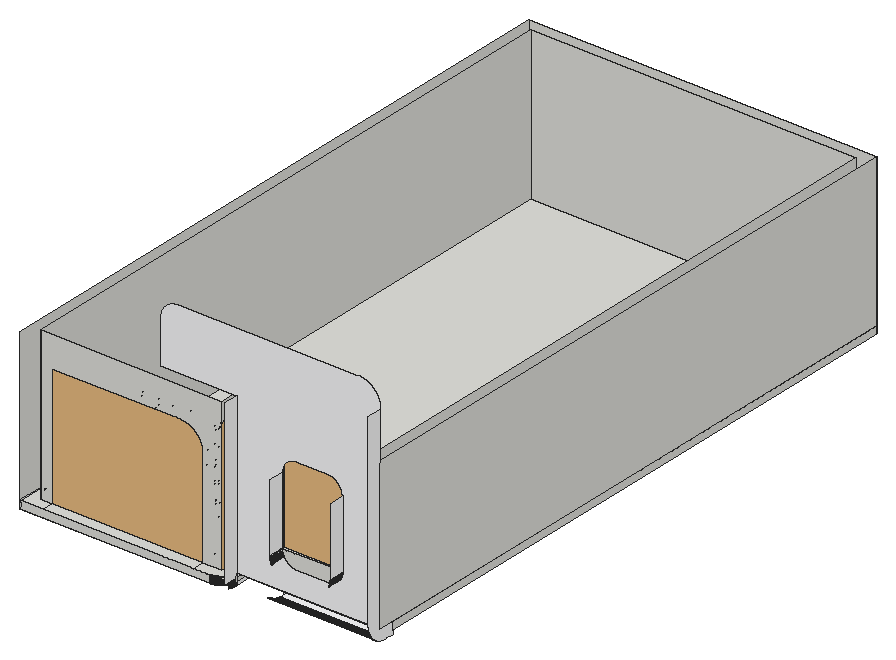
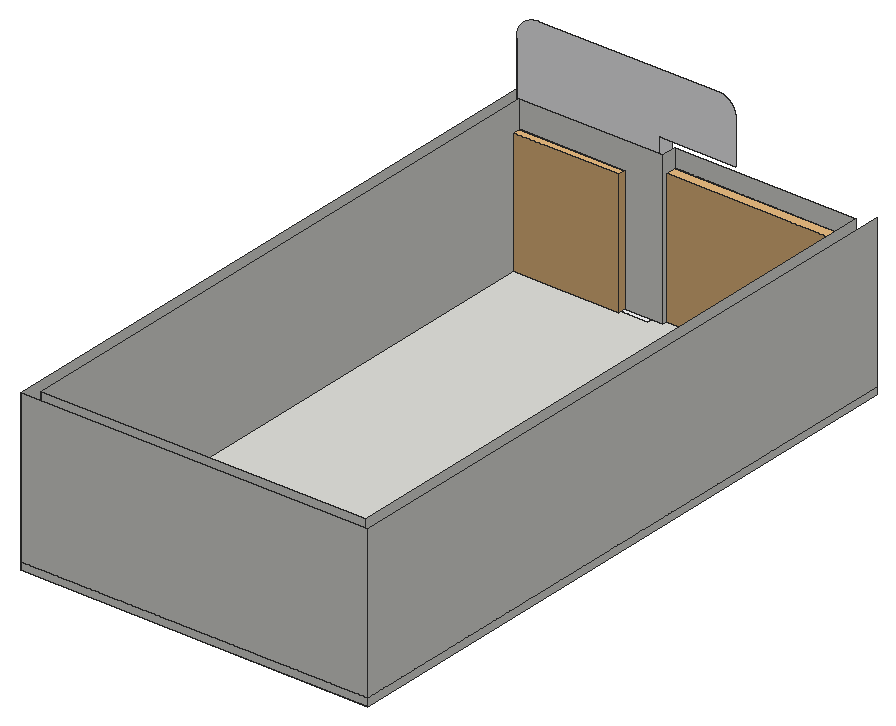
# SketchUp Ruby script. Lengths in inches.
U = 1.inch
M = Sketchup.active_model
def pt(a) = Geom::Point3d.new(a.map { |v| v * U })
def face(e, loops, mat)
  f = e.add_face(loops[0].map { |a| pt(a) })
  loops[1..].each { |l| e.add_face(l.map { |a| pt(a) }).erase! }
  f.material = f.back_material = mat if mat
  f
end
# faces: each face lists its corners as indices into pts; further lists are holes
def faces(e, pts, list, mat = nil) = list.each { |f| face(e, (f[0].is_a?(Array) ? f : [f]).map { |l| l.map { |i| pts[i] } }, mat) }
# xy, xz, yz: faces in a plane at the given z, y or x. An outline is a flat list of corners, or four numbers for a rectangle; further outlines are holes
def ring(l) = l.size == 4 ? [[l[0], l[1]], [l[2], l[1]], [l[2], l[3]], [l[0], l[3]]] : l.each_slice(2).to_a
def flat(e, list, mat, &to3) = list.each { |f| face(e, (f[0].is_a?(Array) ? f : [f]).map { |l| ring(l).map { |u, v| to3.(u, v) } }, mat) }
def xy(e, z, list, mat = nil) = flat(e, list, mat) { |x, y| [x, y, z] }
def xz(e, y, list, mat = nil) = flat(e, list, mat) { |x, z| [x, y, z] }
def yz(e, x, list, mat = nil) = flat(e, list, mat) { |y, z| [x, y, z] }
def lines(e, pts, list) = list.each { |a, b| e.add_line(pt(pts[a]), pt(pts[b])) }
# prism: a flat outline (further loops are holes) pulled along v
def prism(e, loops, v, mat = nil)
  f = face(e, loops, mat); d = Geom::Vector3d.new(v.map { |x| x * U })
  f.pushpull(f.normal.samedirection?(d) ? d.length : -d.length)
end
def box(e, o, s, mat = nil) = prism(e, [[o, [o[0] + s[0], o[1], o[2]], [o[0] + s[0], o[1] + s[1], o[2]], [o[0], o[1] + s[1], o[2]]]], [0, 0, s[2]], mat)
def at(x, y, z, deg = 0) = Geom::Transformation.translation(pt([x, y, z])) * Geom::Transformation.rotation(ORIGIN, Z_AXIS, deg.degrees)
def axes(o, x, y, z) = Geom::Transformation.new([*x, 0, *y, 0, *z, 0, *pt(o).to_a, 1])
def part(name) = M.definitions.add(name)
# library, detail: a bought-in or finely detailed component or shape, given as its bounding box
def library(name, o, s) = part(name).tap { |d| box(d.entities, o, s) }
def detail(e, o, s) = box(e.add_group.entities, o, s)
def put(e, d, t, mat = nil) = e.add_instance(d, t).tap { |i| i.material = mat if mat }
def group(e, t, mat = nil) = e.add_group.tap { |g| g.transformation = t; g.material = mat if mat }.entities
root = M.entities
M.materials.add("[Quartz Light Grey]").color = [251, 251, 252]
M.materials.add("[Wood Veneer 01]").color = [84, 56, 37]
c1 = library("Curtains",[0,0,0],[121.73,8.19,117.22])
c2 = library("Group\#9",[0,-3,0],[48,3,66])
c3 = library("Curtain assembly",[0,0,0],[57.48,5.46,98.43])
xy(root,117,[[228,288.77,312,289],[228,289,312,295]],"[Quartz Light Grey]")
xy(root,117.01,[[228,288.29,312,288.53]],"[Quartz Light Grey]")
xy(root,126,[[36,271,36,775,312,775,312,283,198,283,198,271,174,271,174,280,189,280,189,292,303,292,303,766,45,766,45,280,54,280,54,271]])
xy(root,126,[[198,283,312,295]],"[Quartz Light Grey]")
xy(root,156,[[234,283,282,292]])
xz(root,280,[[45,126,45,246,189,246,189,126,174,126,174,204.4,173.99,204.61,173.96,205.21,173.94,205.41,173.93,205.61,173.91,205.81,173.89,206.02,173.86,206.22,173.84,206.42,173.75,207.02,173.71,207.21,173.55,208.01,173.5,208.2,173.45,208.4,173.4,208.59,173.35,208.79,173.3,208.98,173.24,209.18,173.18,209.37,173.12,209.5625,173.06,209.75,172.99,209.95,172.92,210.14,172.85,210.32,172.71,210.7,172.63,210.89,172.55,211.07,172.47,211.26,172.39,211.44,172.3,211.63,172.22,211.81,171.95,212.35,171.75,212.71,171.66,212.88,171.55,213.06,171.35,213.4,171.24,213.58,171.02,213.92,170.91,214.08,170.8,214.25,170.68,214.42,170.5625,214.58,170.44,214.74,170.32,214.9,170.2,215.0625,170.07,215.22,169.95,215.38,169.82,215.54,169.6875,215.69,169.56,215.84,169.42,215.99,169.29,216.14,169.15,216.29,169.01,216.4375,168.87,216.58,168.73,216.73,168.58,216.87,168.4375,217.01,168.29,217.15,168.14,217.29,167.99,217.42,167.84,217.56,167.69,217.6875,167.54,217.82,167.38,217.95,167.22,218.07,167.0625,218.2,166.9,218.32,166.74,218.44,166.58,218.5625,166.42,218.68,166.25,218.8,166.08,218.91,165.92,219.02,165.58,219.24,165.4,219.35,165.06,219.55,164.88,219.66,164.71,219.75,164.35,219.95,163.81,220.22,163.63,220.3,163.44,220.39,163.26,220.47,163.07,220.55,162.89,220.63,162.7,220.71,162.32,220.85,162.14,220.92,161.95,220.99,161.75,221.06,161.5625,221.12,161.37,221.18,161.18,221.24,160.98,221.3,160.79,221.35,160.59,221.4,160.4,221.45,160.2,221.5,160.01,221.55,159.21,221.71,159.02,221.75,158.42,221.84,158.22,221.86,158.02,221.89,157.81,221.91,157.61,221.93,157.41,221.94,157.21,221.96,156.61,221.99,156.4,222,54,222,54,126]])
xz(root,283,[[[198,126,312,246],[234,156,234,210.3125,234.01,210.47,234.02,210.63,234.03,210.78,234.05,211.1,234.07,211.25,234.08,211.41,234.1,211.57,234.125,211.72,234.15,211.88,234.17,212.03,234.2,212.1875,234.23,212.34,234.26,212.49,234.3,212.65,234.33,212.8,234.37,212.95,234.41,213.11,234.49,213.41,234.64,213.86,234.6875,214.01,234.74,214.15,234.8,214.3,234.85,214.45,234.91,214.59,234.97,214.74,235.04,214.88,235.1,215.02,235.17,215.17,235.45,215.73,235.53,215.86,235.61,216,235.6875,216.14,235.77,216.27,235.85,216.4,235.9375,216.54,236.02,216.67,236.2,216.93,236.29,217.05,236.38,217.18,236.48,217.31,236.58,217.43,236.67,217.55,236.77,217.67,236.98,217.91,237.08,218.03,237.1875,218.15,237.3,218.26,237.4,218.375,237.51,218.49,237.625,218.6,237.74,218.7,237.85,218.8125,237.97,218.92,238.09,219.02,238.33,219.23,238.45,219.33,238.57,219.42,238.69,219.52,238.82,219.62,238.95,219.71,239.07,219.8,239.33,219.98,239.46,220.0625,239.6,220.15,239.73,220.23,239.86,220.3125,240,220.39,240.14,220.47,240.27,220.55,240.83,220.83,240.98,220.9,241.12,220.96,241.26,221.03,241.41,221.09,241.55,221.15,241.7,221.2,241.85,221.26,241.99,221.3125,242.14,221.36,242.59,221.51,242.89,221.59,243.05,221.63,243.2,221.67,243.35,221.7,243.51,221.74,243.66,221.77,243.8125,221.8,243.97,221.83,244.12,221.85,244.28,221.875,244.43,221.9,244.59,221.92,244.75,221.93,244.9,221.95,245.22,221.97,245.37,221.98,245.53,221.99,245.6875,222,270.3125,222,270.47,221.99,270.63,221.98,270.78,221.97,271.1,221.95,271.25,221.93,271.41,221.92,271.57,221.9,271.72,221.875,271.88,221.85,272.03,221.83,272.1875,221.8,272.34,221.77,272.49,221.74,272.65,221.7,272.8,221.67,272.95,221.63,273.11,221.59,273.41,221.51,273.86,221.36,274.01,221.3125,274.15,221.26,274.3,221.2,274.45,221.15,274.59,221.09,274.74,221.03,274.88,220.96,275.02,220.9,275.17,220.83,275.73,220.55,275.86,220.47,276,220.39,276.14,220.3125,276.27,220.23,276.4,220.15,276.54,220.0625,276.67,219.98,276.93,219.8,277.05,219.71,277.18,219.62,277.31,219.52,277.43,219.42,277.55,219.33,277.67,219.23,277.91,219.02,278.03,218.92,278.15,218.8125,278.26,218.7,278.375,218.6,278.49,218.49,278.6,218.375,278.7,218.26,278.8125,218.15,278.92,218.03,279.02,217.91,279.23,217.67,279.33,217.55,279.42,217.43,279.52,217.31,279.62,217.18,279.71,217.05,279.8,216.93,279.98,216.67,280.0625,216.54,280.15,216.4,280.23,216.27,280.3125,216.14,280.39,216,280.47,215.86,280.55,215.73,280.83,215.17,280.9,215.02,280.96,214.88,281.03,214.74,281.09,214.59,281.15,214.45,281.2,214.3,281.26,214.15,281.3125,214.01,281.36,213.86,281.51,213.41,281.59,213.11,281.63,212.95,281.67,212.8,281.7,212.65,281.74,212.49,281.77,212.34,281.8,212.1875,281.83,212.03,281.85,211.88,281.875,211.72,281.9,211.57,281.92,211.41,281.93,211.25,281.95,211.1,281.97,210.78,281.98,210.63,281.99,210.47,282,210.3125,282,156]]])
xz(root,283,[[[198,126,198,252,138,252,138,286.37,138.02,286.73,138.03,286.92,138.04,287.1,138.08,287.46,138.1,287.65,138.14,288.01,138.23,288.55,138.43,289.45,138.53,289.8,138.58,289.98,138.63,290.15,138.69,290.33,138.74,290.5,138.8,290.67,138.87,290.85,138.93,291.02,139,291.1875,139.07,291.36,139.14,291.53,139.21,291.69,139.29,291.86,139.36,292.03,139.44,292.19,139.53,292.36,139.61,292.52,139.79,292.84,139.875,293,139.97,293.16,140.0625,293.31,140.16,293.47,140.36,293.78,140.46,293.93,140.57,294.08,140.67,294.23,140.89,294.52,141.01,294.67,141.12,294.81,141.24,294.95,141.35,295.09,141.47,295.23,141.6,295.37,141.72,295.5,141.84,295.64,142.36,296.16,142.5,296.28,142.63,296.4,142.77,296.53,142.91,296.65,143.05,296.76,143.19,296.88,143.33,296.99,143.48,297.11,143.77,297.33,143.92,297.43,144.07,297.54,144.22,297.64,144.53,297.84,144.69,297.9375,144.84,298.03,145,298.125,145.16,298.21,145.48,298.39,145.64,298.47,145.81,298.56,145.97,298.64,146.14,298.71,146.31,298.79,146.47,298.86,146.64,298.93,146.8125,299,146.98,299.07,147.15,299.13,147.33,299.2,147.5,299.26,147.67,299.31,147.85,299.37,148.02,299.42,148.2,299.47,148.55,299.57,149.45,299.77,149.99,299.86,150.35,299.9,150.54,299.92,150.9,299.96,151.08,299.97,151.27,299.98,151.63,300,294.24,300,294.47,299.99,294.71,299.99,294.94,299.98,295.18,299.96,295.41,299.94,295.65,299.92,295.88,299.9,296.12,299.875,296.35,299.85,296.58,299.8125,296.82,299.78,297.28,299.7,297.51,299.65,297.74,299.61,297.97,299.56,298.2,299.5,298.43,299.45,298.66,299.39,298.89,299.32,299.11,299.26,299.34,299.19,299.5625,299.12,299.79,299.04,300.01,298.97,300.23,298.89,300.45,298.8,300.67,298.72,301.11,298.54,301.32,298.44,301.54,298.35,301.75,298.25,301.96,298.14,302.17,298.04,302.59,297.82,302.8,297.7,303,297.59,303.4,297.35,303.61,297.22,303.8,297.1,304,296.97,304.2,296.83,304.39,296.7,304.58,296.5625,304.77,296.42,304.96,296.28,305.14,296.14,305.33,295.99,305.51,295.84,305.69,295.6875,305.87,295.53,306.04,295.375,306.22,295.22,306.39,295.06,306.56,294.89,306.73,294.73,306.89,294.56,307.06,294.39,307.22,294.22,307.375,294.04,307.53,293.87,307.6875,293.69,307.84,293.51,307.99,293.33,308.14,293.14,308.28,292.96,308.42,292.77,308.5625,292.58,308.7,292.39,308.83,292.2,308.97,292,309.1,291.8,309.22,291.61,309.35,291.4,309.59,291,309.7,290.8,309.82,290.59,310.04,290.17,310.14,289.96,310.25,289.75,310.35,289.54,310.44,289.32,310.54,289.11,310.72,288.67,310.8,288.45,310.89,288.23,310.97,288.01,311.04,287.79,311.12,287.5625,311.19,287.34,311.26,287.11,311.32,286.89,311.39,286.66,311.45,286.43,311.5,286.2,311.56,285.97,311.61,285.74,311.65,285.51,311.7,285.28,311.78,284.82,311.8125,284.58,311.85,284.35,311.875,284.12,311.9,283.88,311.92,283.65,311.94,283.41,311.96,283.18,311.98,282.94,311.99,282.71,311.99,282.47,312,282.24,312,126],[245.84,144,270.16,144,270.3125,144.01,270.47,144.01,270.63,144.02,270.78,144.03,271.1,144.05,271.25,144.07,271.41,144.08,271.57,144.1,271.72,144.125,271.88,144.15,272.03,144.17,272.1875,144.2,272.34,144.23,272.49,144.26,272.65,144.3,272.8,144.33,272.95,144.37,273.11,144.41,273.26,144.45,273.41,144.5,273.56,144.54,274.01,144.69,274.15,144.74,274.45,144.86,274.59,144.91,274.74,144.98,275.02,145.1,275.17,145.17,275.59,145.38,275.73,145.46,275.86,145.53,276,145.61,276.14,145.6875,276.27,145.77,276.4,145.85,276.54,145.9375,276.67,146.02,276.93,146.2,277.05,146.29,277.18,146.39,277.3,146.48,277.43,146.58,277.55,146.68,277.67,146.77,277.91,146.98,278.03,147.08,278.15,147.1875,278.26,147.3,278.48,147.52,278.6,147.63,278.7,147.74,278.8125,147.86,278.92,147.97,279.02,148.09,279.23,148.33,279.33,148.45,279.42,148.57,279.52,148.7,279.61,148.82,279.71,148.95,279.8,149.07,279.98,149.33,280.0625,149.47,280.15,149.6,280.23,149.73,280.3125,149.87,280.39,150,280.47,150.14,280.55,150.27,280.83,150.83,280.9,150.98,280.96,151.12,281.03,151.26,281.09,151.41,281.15,151.55,281.2,151.7,281.26,151.85,281.3125,151.99,281.36,152.14,281.51,152.59,281.59,152.89,281.63,153.05,281.67,153.2,281.7,153.35,281.74,153.51,281.77,153.66,281.8,153.8125,281.83,153.97,281.85,154.12,281.875,154.28,281.9,154.43,281.92,154.59,281.93,154.75,281.95,154.9,281.97,155.22,281.98,155.37,281.99,155.53,282,155.6875,282,210.3125,281.99,210.47,281.98,210.63,281.97,210.78,281.95,211.1,281.93,211.25,281.92,211.41,281.9,211.57,281.875,211.72,281.85,211.88,281.83,212.03,281.8,212.1875,281.77,212.34,281.74,212.49,281.7,212.65,281.67,212.8,281.63,212.95,281.59,213.11,281.51,213.41,281.36,213.86,281.3125,214.01,281.26,214.15,281.2,214.3,281.15,214.45,281.09,214.59,281.03,214.74,280.96,214.88,280.9,215.02,280.83,215.17,280.55,215.73,280.47,215.86,280.39,216,280.3125,216.14,280.23,216.27,280.15,216.4,280.0625,216.54,279.98,216.67,279.8,216.93,279.71,217.05,279.62,217.18,279.52,217.31,279.42,217.43,279.33,217.55,279.23,217.67,279.02,217.91,278.92,218.03,278.8125,218.15,278.7,218.26,278.6,218.375,278.49,218.49,278.375,218.6,278.26,218.7,278.15,218.8125,278.03,218.92,277.91,219.02,277.67,219.23,277.55,219.33,277.43,219.42,277.31,219.52,277.18,219.62,277.05,219.71,276.93,219.8,276.67,219.98,276.54,220.0625,276.4,220.15,276.27,220.23,276.14,220.3125,276,220.39,275.86,220.47,275.73,220.55,275.17,220.83,275.02,220.9,274.88,220.96,274.74,221.03,274.59,221.09,274.45,221.15,274.3,221.2,274.15,221.26,274.01,221.3125,273.86,221.36,273.41,221.51,273.11,221.59,272.95,221.63,272.8,221.67,272.65,221.7,272.49,221.74,272.34,221.77,272.1875,221.8,272.03,221.83,271.88,221.85,271.72,221.875,271.57,221.9,271.41,221.92,271.25,221.93,271.1,221.95,270.78,221.97,270.63,221.98,270.47,221.99,270.3125,222,245.6875,222,245.53,221.99,245.37,221.98,245.22,221.97,244.9,221.95,244.75,221.93,244.59,221.92,244.43,221.9,244.28,221.875,244.12,221.85,243.97,221.83,243.8125,221.8,243.66,221.77,243.51,221.74,243.35,221.7,243.2,221.67,243.05,221.63,242.89,221.59,242.59,221.51,242.14,221.36,241.99,221.3125,241.85,221.26,241.7,221.2,241.55,221.15,241.41,221.09,241.26,221.03,241.12,220.96,240.98,220.9,240.83,220.83,240.27,220.55,240.14,220.47,240,220.39,239.86,220.3125,239.73,220.23,239.6,220.15,239.46,220.0625,239.33,219.98,239.07,219.8,238.95,219.71,238.82,219.62,238.69,219.52,238.57,219.42,238.45,219.33,238.33,219.23,238.09,219.02,237.97,218.92,237.85,218.8125,237.74,218.7,237.625,218.6,237.51,218.49,237.4,218.375,237.3,218.26,237.1875,218.15,237.08,218.03,236.98,217.91,236.77,217.67,236.67,217.55,236.58,217.43,236.48,217.31,236.38,217.18,236.29,217.05,236.2,216.93,236.02,216.67,235.9375,216.54,235.85,216.4,235.77,216.27,235.6875,216.14,235.61,216,235.53,215.86,235.45,215.73,235.17,215.17,235.1,215.02,235.04,214.88,234.97,214.74,234.91,214.59,234.85,214.45,234.8,214.3,234.74,214.15,234.6875,214.01,234.64,213.86,234.49,213.41,234.41,213.11,234.37,212.95,234.33,212.8,234.3,212.65,234.26,212.49,234.23,212.34,234.2,212.1875,234.17,212.03,234.15,211.88,234.125,211.72,234.1,211.57,234.08,211.41,234.07,211.25,234.05,211.1,234.03,210.78,234.02,210.63,234.01,210.47,234,210.3125,234,155.6875,234.01,155.53,234.02,155.37,234.03,155.22,234.05,154.9,234.07,154.75,234.08,154.59,234.1,154.43,234.125,154.28,234.15,154.12,234.17,153.97,234.2,153.8125,234.23,153.66,234.26,153.51,234.3,153.35,234.33,153.2,234.37,153.05,234.41,152.89,234.49,152.59,234.64,152.14,234.6875,151.99,234.74,151.85,234.8,151.7,234.85,151.55,234.91,151.41,234.97,151.26,235.04,151.12,235.1,150.98,235.17,150.83,235.45,150.27,235.53,150.14,235.61,150,235.6875,149.87,235.77,149.73,235.85,149.6,235.9375,149.47,236.02,149.33,236.2,149.07,236.29,148.95,236.39,148.82,236.48,148.7,236.58,148.57,236.67,148.45,236.77,148.33,236.98,148.09,237.08,147.97,237.1875,147.86,237.3,147.74,237.4,147.63,237.52,147.52,237.74,147.3,237.85,147.1875,237.97,147.08,238.09,146.98,238.33,146.77,238.45,146.68,238.57,146.58,238.7,146.48,238.82,146.39,238.95,146.29,239.07,146.2,239.33,146.02,239.46,145.9375,239.6,145.85,239.73,145.77,239.86,145.6875,240,145.61,240.14,145.53,240.27,145.46,240.41,145.38,240.83,145.17,240.98,145.1,241.26,144.98,241.41,144.91,241.55,144.86,241.85,144.74,241.99,144.69,242.44,144.54,242.59,144.5,242.74,144.45,242.89,144.41,243.05,144.37,243.2,144.33,243.35,144.3,243.51,144.26,243.66,144.23,243.8125,144.2,243.97,144.17,244.12,144.15,244.28,144.125,244.43,144.1,244.59,144.08,244.75,144.07,244.9,144.05,245.22,144.03,245.37,144.02,245.53,144.01,245.6875,144.01]]],"[Quartz Light Grey]")
xz(root,292,[[[189,126,303,246],[234,156,282,156,282,210.3125,281.99,210.47,281.98,210.63,281.97,210.78,281.95,211.1,281.93,211.25,281.92,211.41,281.9,211.57,281.875,211.72,281.85,211.88,281.83,212.03,281.8,212.1875,281.77,212.34,281.74,212.49,281.7,212.65,281.67,212.8,281.63,212.95,281.59,213.11,281.51,213.41,281.36,213.86,281.3125,214.01,281.26,214.15,281.2,214.3,281.15,214.45,281.09,214.59,281.03,214.74,280.96,214.88,280.9,215.02,280.83,215.17,280.55,215.73,280.47,215.86,280.39,216,280.3125,216.14,280.23,216.27,280.15,216.4,280.0625,216.54,279.98,216.67,279.8,216.93,279.71,217.05,279.62,217.18,279.52,217.31,279.42,217.43,279.33,217.55,279.23,217.67,279.02,217.91,278.92,218.03,278.8125,218.15,278.7,218.26,278.6,218.375,278.49,218.49,278.375,218.6,278.26,218.7,278.15,218.8125,278.03,218.92,277.91,219.02,277.67,219.23,277.55,219.33,277.43,219.42,277.31,219.52,277.18,219.62,277.05,219.71,276.93,219.8,276.67,219.98,276.54,220.0625,276.4,220.15,276.27,220.23,276.14,220.3125,276,220.39,275.86,220.47,275.73,220.55,275.17,220.83,275.02,220.9,274.88,220.96,274.74,221.03,274.59,221.09,274.45,221.15,274.3,221.2,274.15,221.26,274.01,221.3125,273.86,221.36,273.41,221.51,273.11,221.59,272.95,221.63,272.8,221.67,272.65,221.7,272.49,221.74,272.34,221.77,272.1875,221.8,272.03,221.83,271.88,221.85,271.72,221.875,271.57,221.9,271.41,221.92,271.25,221.93,271.1,221.95,270.78,221.97,270.63,221.98,270.47,221.99,270.3125,222,245.6875,222,245.53,221.99,245.37,221.98,245.22,221.97,244.9,221.95,244.75,221.93,244.59,221.92,244.43,221.9,244.28,221.875,244.12,221.85,243.97,221.83,243.8125,221.8,243.66,221.77,243.51,221.74,243.35,221.7,243.2,221.67,243.05,221.63,242.89,221.59,242.59,221.51,242.14,221.36,241.99,221.3125,241.85,221.26,241.7,221.2,241.55,221.15,241.41,221.09,241.26,221.03,241.12,220.96,240.98,220.9,240.83,220.83,240.27,220.55,240.14,220.47,240,220.39,239.86,220.3125,239.73,220.23,239.6,220.15,239.46,220.0625,239.33,219.98,239.07,219.8,238.95,219.71,238.82,219.62,238.69,219.52,238.57,219.42,238.45,219.33,238.33,219.23,238.09,219.02,237.97,218.92,237.85,218.8125,237.74,218.7,237.625,218.6,237.51,218.49,237.4,218.375,237.3,218.26,237.1875,218.15,237.08,218.03,236.98,217.91,236.77,217.67,236.67,217.55,236.58,217.43,236.48,217.31,236.38,217.18,236.29,217.05,236.2,216.93,236.02,216.67,235.9375,216.54,235.85,216.4,235.77,216.27,235.6875,216.14,235.61,216,235.53,215.86,235.45,215.73,235.17,215.17,235.1,215.02,235.04,214.88,234.97,214.74,234.91,214.59,234.85,214.45,234.8,214.3,234.74,214.15,234.6875,214.01,234.64,213.86,234.49,213.41,234.41,213.11,234.37,212.95,234.33,212.8,234.3,212.65,234.26,212.49,234.23,212.34,234.2,212.1875,234.17,212.03,234.15,211.88,234.125,211.72,234.1,211.57,234.08,211.41,234.07,211.25,234.05,211.1,234.03,210.78,234.02,210.63,234.01,210.47,234,210.3125]]])
xz(root,295,[[226,115,228,117],[198,117,312,126]],"[Quartz Light Grey]")
xz(root,766,[[45,126,303,246]])
xz(root,775,[[36,126,312,246]])
yz(root,36,[[271,126,775,246]])
yz(root,45,[[280,126,766,246]])
yz(root,189,[[280,126,292,246]])
yz(root,198,[[282.6875,117,282.84,123],[282.84,117,283,123],[283,117,295,123],[271,123,271,252,283,252,283,126,295,126,295,123]],"[Quartz Light Grey]")
yz(root,234,[[283,156,292,210]])
yz(root,234,[[271,155.6875,283,155.84],[271,155.84,283,156],[271,156,283,210]],"[Quartz Light Grey]")
yz(root,282,[[283,156,292,210]])
yz(root,282,[[271,155.6875,283,155.84],[271,155.84,283,156],[271,156,283,210]],"[Quartz Light Grey]")
yz(root,303,[[292,126,766,246]])
yz(root,312,[[283,126,775,246]])
yz(root,312,[[288.77,117,295,117,295,126,283,126,283,282,271,282,271,134.77,271.01,134.53,271.01,134.29,271.02,134.06,271.04,133.82,271.06,133.59,271.08,133.35,271.1,133.12,271.125,132.89,271.15,132.65,271.1875,132.42,271.22,132.19,271.26,131.95,271.3,131.72,271.35,131.49,271.39,131.26,271.44,131.03,271.5,130.8,271.55,130.57,271.61,130.34,271.68,130.12,271.74,129.89,271.81,129.66,271.88,129.4375,271.96,129.22,272.03,128.99,272.11,128.77,272.2,128.55,272.28,128.33,272.37,128.11,272.46,127.9,272.56,127.68,272.65,127.46,272.75,127.25,272.86,127.04,272.96,126.83,273.18,126.41,273.3,126.21,273.41,126,273.65,125.6,273.78,125.4,273.9,125.2,274.03,125,274.17,124.81,274.3,124.61,274.4375,124.42,274.58,124.23,274.72,124.04,274.86,123.86,275.01,123.67,275.16,123.49,275.3125,123.31,275.47,123.13,275.625,122.96,275.78,122.78,275.94,122.61,276.11,122.44,276.27,122.27,276.44,122.11,276.61,121.94,276.78,121.78,276.96,121.625,277.13,121.47,277.31,121.3125,277.49,121.16,277.67,121.01,277.86,120.86,278.04,120.72,278.23,120.58,278.42,120.4375,278.61,120.3,278.81,120.17,279,120.03,279.2,119.9,279.4,119.78,279.6,119.65,280,119.41,280.21,119.3,280.41,119.18,280.83,118.96,281.04,118.86,281.25,118.75,281.46,118.65,281.68,118.56,281.9,118.46,282.11,118.37,282.33,118.28,282.55,118.2,282.77,118.11,282.99,118.03,283.22,117.96,283.4375,117.88,283.66,117.81,283.89,117.74,284.12,117.68,284.34,117.61,284.57,117.55,284.8,117.5,285.03,117.44,285.26,117.39,285.49,117.35,285.72,117.3,285.95,117.26,286.19,117.22,286.42,117.1875,286.65,117.15,286.89,117.125,287.12,117.1,287.35,117.08,287.59,117.06,287.82,117.04,288.06,117.02,288.29,117.01,288.53,117.01]],"[Quartz Light Grey]")
p = [[196.47,277.14,117],[196.39,277,117],[196.39,277,123],[196.47,277.14,123],[196.55,277.27,117],[196.55,277.27,123],
  [196.62,277.41,117],[196.62,277.41,123],[196.69,277.55,117],[196.69,277.55,123],[196.76,277.69,117],[196.76,277.69,123],
  [196.83,277.83,117],[196.83,277.83,123],[196.9,277.98,117],[196.9,277.98,123],[196.96,278.12,117],[196.96,278.12,123],
  [197.03,278.26,117],[197.03,278.26,123],[197.09,278.41,117],[197.09,278.41,123],[197.15,278.55,117],[197.15,278.55,123],
  [197.2,278.7,117],[197.2,278.7,123],[197.26,278.85,117],[197.26,278.85,123],[197.3125,278.99,117],[197.3125,278.99,123],
  [197.36,279.14,117],[197.36,279.14,123],[197.41,279.29,117],[197.41,279.29,123],[197.46,279.44,117],[197.46,279.44,123],
  [197.51,279.59,117],[197.51,279.59,123],[197.55,279.74,117],[197.55,279.74,123],[197.59,279.89,117],[197.59,279.89,123],
  [197.63,280.05,117],[197.63,280.05,123],[197.67,280.2,117],[197.67,280.2,123],[197.7,280.35,117],[197.7,280.35,123],
  [197.74,280.51,117],[197.74,280.51,123],[197.77,280.66,117],[197.77,280.66,123],[197.8,280.8125,117],[197.8,280.8125,123],
  [197.83,280.97,117],[197.83,280.97,123],[197.85,281.12,117],[197.85,281.12,123],[197.875,281.28,117],[197.875,281.28,123],
  [197.9,281.43,117],[197.9,281.43,123],[197.92,281.59,117],[197.92,281.59,123],[197.93,281.75,117],[197.93,281.75,123],
  [197.95,281.9,117],[197.95,281.9,123],[197.96,282.06,117],[197.96,282.06,123],[197.97,282.22,117],[197.97,282.22,123],
  [197.98,282.37,117],[197.98,282.37,123],[197.99,282.53,117],[197.99,282.53,123],[198,282.6875,117],[198,282.6875,123],
  [312,287.82,117.04],[312,287.59,117.06],[228,287.59,117.06],[228,287.82,117.04],[312,288.06,117.02],[228,288.06,117.02],
  [312,288.29,117.01],[228,288.29,117.01],[312,288.77,117],[312,288.53,117.01],[228,288.53,117.01],[228,288.77,117],
  [312,286.89,117.125],[312,286.65,117.15],[228,286.65,117.15],[228,286.89,117.125],[312,287.12,117.1],[228,287.12,117.1],
  [312,287.35,117.08],[228,287.35,117.08],[312,286.19,117.22],[312,285.95,117.26],[228,285.95,117.26],[228,286.19,117.22],
  [312,286.42,117.1875],[228,286.42,117.1875],[312,285.49,117.35],[312,285.26,117.39],[228,285.26,117.39],[228,285.49,117.35],
  [312,285.72,117.3],[228,285.72,117.3],[312,285.03,117.44],[312,284.8,117.5],[228,284.8,117.5],[228,285.03,117.44],
  [312,284.57,117.55],[228,284.57,117.55],[312,284.34,117.61],[312,284.12,117.68],[228,284.12,117.68],[228,284.34,117.61],
  [312,283.89,117.74],[312,283.66,117.81],[228,283.66,117.81],[228,283.89,117.74],[312,283.4375,117.88],[228,283.4375,117.88],
  [312,283.22,117.96],[228,283.22,117.96],[312,282.99,118.03],[312,282.77,118.11],[228,282.77,118.11],[228,282.99,118.03],
  [312,282.55,118.2],[228,282.55,118.2],[312,282.33,118.28],[228,282.33,118.28],[312,282.11,118.37],[228,282.11,118.37],
  [312,281.9,118.46],[228,281.9,118.46],[312,281.68,118.56],[228,281.68,118.56],[312,281.46,118.65],[228,281.46,118.65],
  [312,281.25,118.75],[228,281.25,118.75],[312,281.04,118.86],[228,281.04,118.86],[312,280.83,118.96],[228,280.83,118.96],
  [312,280.62,119.07],[228,280.62,119.07],[312,280.41,119.18],[228,280.41,119.18],[312,280.21,119.3],[228,280.21,119.3],
  [312,280,119.41],[228,280,119.41],[312,279.8,119.53],[228,279.8,119.53],[312,279.6,119.65],[228,279.6,119.65],
  [312,279.4,119.78],[228,279.4,119.78],[312,279.2,119.9],[228,279.2,119.9],[312,279,120.03],[228,279,120.03],
  [312,278.81,120.17],[228,278.81,120.17],[312,278.61,120.3],[228,278.61,120.3],[312,278.42,120.4375],[228,278.42,120.4375],
  [312,278.23,120.58],[228,278.23,120.58],[312,278.04,120.72],[228,278.04,120.72],[312,277.86,120.86],[228,277.86,120.86],
  [312,277.67,121.01],[228,277.67,121.01],[312,277.49,121.16],[228,277.49,121.16],[312,277.31,121.3125],[228,277.31,121.3125],
  [312,277.13,121.47],[228,277.13,121.47],[312,276.96,121.625],[228,276.96,121.625],[235.45,283,150.27],[235.38,283,150.41],
  [235.38,271,150.41],[235.45,271,150.27],[280.62,283,150.41],[280.55,283,150.27],[280.55,271,150.27],[280.62,271,150.41],
  [235.31,283,150.55],[235.31,271,150.55],[280.69,283,150.55],[280.69,271,150.55],[235.24,283,150.69],[235.24,271,150.69],
  [280.76,283,150.69],[280.76,271,150.69],[235.17,283,150.83],[235.17,271,150.83],[280.83,283,150.83],[280.83,271,150.83],
  [235.1,283,150.98],[235.1,271,150.98],[280.9,283,150.98],[280.9,271,150.98],[235.04,283,151.12],[235.04,271,151.12],
  [280.96,283,151.12],[280.96,271,151.12],[234.97,283,151.26],[234.97,271,151.26],[281.03,283,151.26],[281.03,271,151.26],
  [234.91,283,151.41],[234.91,271,151.41],[281.09,283,151.41],[281.09,271,151.41],[234.85,283,151.55],[234.85,271,151.55],
  [281.15,283,151.55],[281.15,271,151.55],[234.8,283,151.7],[234.8,271,151.7],[281.2,283,151.7],[281.2,271,151.7],
  [234.74,283,151.85],[234.74,271,151.85],[281.26,283,151.85],[281.26,271,151.85],[234.6875,283,151.99],[234.6875,271,151.99],
  [281.3125,283,151.99],[281.3125,271,151.99],[234.64,283,152.14],[234.64,271,152.14],[281.36,283,152.14],[281.36,271,152.14],
  [234.59,283,152.29],[234.59,271,152.29],[281.41,283,152.29],[281.41,271,152.29],[234.54,283,152.44],[234.54,271,152.44],
  [281.46,283,152.44],[281.46,271,152.44],[234.49,283,152.59],[234.49,271,152.59],[281.51,283,152.59],[281.51,271,152.59],
  [234.45,283,152.74],[234.45,271,152.74],[281.55,283,152.74],[281.55,271,152.74],[234.41,283,152.89],[234.41,271,152.89],
  [281.59,283,152.89],[281.59,271,152.89],[234.37,283,153.05],[234.37,271,153.05],[281.63,283,153.05],[281.63,271,153.05],
  [234.33,283,153.2],[234.33,271,153.2],[281.67,283,153.2],[281.67,271,153.2],[234.3,283,153.35],[234.3,271,153.35],
  [281.7,283,153.35],[281.7,271,153.35],[234.26,283,153.51],[234.26,271,153.51],[281.74,283,153.51],[281.74,271,153.51],
  [234.23,283,153.66],[234.23,271,153.66],[281.77,283,153.66],[281.77,271,153.66],[234.2,283,153.8125],[234.2,271,153.8125],
  [281.8,283,153.8125],[281.8,271,153.8125],[234.17,283,153.97],[234.17,271,153.97],[281.83,283,153.97],[281.83,271,153.97],
  [234.15,283,154.12],[234.15,271,154.12],[281.85,283,154.12],[281.85,271,154.12],[234.125,283,154.28],[234.125,271,154.28],
  [281.875,283,154.28],[281.875,271,154.28],[234.1,283,154.43],[234.1,271,154.43],[281.9,283,154.43],[281.9,271,154.43],
  [234.08,283,154.59],[234.08,271,154.59],[281.92,283,154.59],[281.92,271,154.59],[234.07,283,154.75],[234.07,271,154.75],
  [281.93,283,154.75],[281.93,271,154.75],[234.05,283,154.9],[234.05,271,154.9],[281.95,283,154.9],[281.95,271,154.9],
  [234.04,283,155.06],[234.04,271,155.06],[281.96,283,155.06],[281.96,271,155.06],[234.03,283,155.22],[234.03,271,155.22],
  [281.97,283,155.22],[281.97,271,155.22],[234.02,283,155.37],[234.02,271,155.37],[281.98,283,155.37],[281.98,271,155.37],
  [234.01,283,155.53],[234.01,271,155.53],[281.99,283,155.53],[281.99,271,155.53],[234,283,155.6875],[234,271,155.6875],
  [282,283,155.6875],[282,271,155.6875],[312,283.08,126.08],[303,283.08,126.08]]
faces(root,p,[[0,1,2,3],[4,0,3,5],[6,4,5,7],[8,6,7,9],[10,8,9,11],[12,10,11,13],[14,12,13,15],[16,14,15,17],
  [18,16,17,19],[20,18,19,21],[22,20,21,23],[24,22,23,25],[26,24,25,27],[28,26,27,29],[30,28,29,31],[32,30,31,33],
  [34,32,33,35],[36,34,35,37],[38,36,37,39],[40,38,39,41],[42,40,41,43],[44,42,43,45],[46,44,45,47],[48,46,47,49],
  [50,48,49,51],[52,50,51,53],[54,52,53,55],[56,54,55,57],[58,56,57,59],[60,58,59,61],[62,60,61,63],[64,62,63,65],
  [66,64,65,67],[68,66,67,69],[70,68,69,71],[72,70,71,73],[74,72,73,75],[76,74,75,77],[78,79,80,81],[82,78,81,83],
  [84,82,83,85],[86,87,88,89],[90,91,92,93],[94,90,93,95],[96,94,95,97],[79,96,97,80],[98,99,100,101],[102,98,101,103],
  [91,102,103,92],[104,105,106,107],[108,104,107,109],[99,108,109,100],[110,111,112,113],[105,110,113,106],[111,114,115,112],[116,117,118,119],
  [114,116,119,115],[120,121,122,123],[117,120,123,118],[121,124,125,122],[124,126,127,125],[128,129,130,131],[126,128,131,127],[129,132,133,130],
  [132,134,135,133],[134,136,137,135],[136,138,139,137],[138,140,141,139],[140,142,143,141],[142,144,145,143],[144,146,147,145],[146,148,149,147],
  [148,150,151,149],[150,152,153,151],[152,154,155,153],[154,156,157,155],[156,158,159,157],[158,160,161,159],[160,162,163,161],[162,164,165,163],
  [164,166,167,165],[166,168,169,167],[168,170,171,169],[170,172,173,171],[172,174,175,173],[174,176,177,175],[176,178,179,177],[178,180,181,179],
  [180,182,183,181],[182,184,185,183],[184,186,187,185],[186,188,189,187],[190,191,192,193],[194,195,196,197],[191,198,199,192],[200,194,197,201],
  [198,202,203,199],[204,200,201,205],[202,206,207,203],[208,204,205,209],[206,210,211,207],[212,208,209,213],[210,214,215,211],[216,212,213,217],
  [214,218,219,215],[220,216,217,221],[218,222,223,219],[224,220,221,225],[222,226,227,223],[228,224,225,229],[226,230,231,227],[232,228,229,233],
  [230,234,235,231],[236,232,233,237],[234,238,239,235],[240,236,237,241],[238,242,243,239],[244,240,241,245],[242,246,247,243],[248,244,245,249],
  [246,250,251,247],[252,248,249,253],[250,254,255,251],[256,252,253,257],[254,258,259,255],[260,256,257,261],[258,262,263,259],[264,260,261,265],
  [262,266,267,263],[268,264,265,269],[266,270,271,267],[272,268,269,273],[270,274,275,271],[276,272,273,277],[274,278,279,275],[280,276,277,281],
  [278,282,283,279],[284,280,281,285],[282,286,287,283],[288,284,285,289],[286,290,291,287],[292,288,289,293],[290,294,295,291],[296,292,293,297],
  [294,298,299,295],[300,296,297,301],[298,302,303,299],[304,300,301,305],[302,306,307,303],[308,304,305,309],[306,310,311,307],[312,308,309,313],
  [310,314,315,311],[316,312,313,317],[314,318,319,315],[320,316,317,321],[318,322,323,319],[324,320,321,325],[322,326,327,323],[328,324,325,329],
  [326,330,331,327],[332,328,329,333],[330,334,335,331],[336,332,333,337]],"[Quartz Light Grey]")
lines(root,p,[[338,339]])
put(root,c1,axes([45,288.19,126],[1.18298,0,0],[0,-1,0],[0,0,0.9]))
put(root,c2,at(234,288,156),"[Wood Veneer 01]")
put(root,c3,axes([219.08,292,126],[1.46,0,0],[0,1,0],[0,0,1]))
g1 = group(root,at(36,271,120))
prism(g1,[[[0,0,0],[0,504,0],[276,504,0],[276,24,0],[162,24,0],[162,12,0],[162,11.84,0],[162,11.6875,0],[161.99,11.53,0],[161.98,11.37,0],[161.97,11.22,0],[161.96,11.06,0],[161.95,10.9,0],[161.93,10.75,0],[161.92,10.59,0],[161.9,10.43,0],[161.875,10.28,0],[161.85,10.12,0],[161.83,9.97,0],[161.8,9.8125,0],[161.77,9.66,0],[161.74,9.51,0],[161.7,9.35,0],[161.67,9.2,0],[161.63,9.05,0],[161.59,8.89,0],[161.55,8.74,0],[161.51,8.59,0],[161.46,8.44,0],[161.41,8.29,0],[161.36,8.14,0],[161.3125,7.99,0],[161.26,7.85,0],[161.2,7.7,0],[161.15,7.55,0],[161.09,7.41,0],[161.03,7.26,0],[160.96,7.12,0],[160.9,6.98,0],[160.83,6.83,0],[160.76,6.69,0],[160.69,6.55,0],[160.62,6.41,0],[160.55,6.27,0],[160.47,6.14,0],[160.39,6,0],[160.3125,5.86,0],[160.23,5.73,0],[160.15,5.6,0],[160.0625,5.46,0],[159.98,5.33,0],[159.89,5.2,0],[159.8,5.07,0],[159.71,4.95,0],[159.62,4.82,0],[159.52,4.69,0],[159.42,4.57,0],[159.33,4.45,0],[159.23,4.33,0],[159.125,4.21,0],[159.02,4.09,0],[158.92,3.97,0],[158.8125,3.85,0],[158.7,3.74,0],[158.6,3.625,0],[158.49,3.51,0],[158.375,3.4,0],[158.26,3.3,0],[158.15,3.1875,0],[158.03,3.08,0],[157.91,2.98,0],[157.79,2.875,0],[157.67,2.77,0],[157.55,2.67,0],[157.43,2.58,0],[157.31,2.48,0],[157.18,2.38,0],[157.05,2.29,0],[156.93,2.2,0],[156.8,2.11,0],[156.67,2.02,0],[156.54,1.9375,0],[156.4,1.85,0],[156.27,1.77,0],[156.14,1.6875,0],[156,1.61,0],[155.86,1.53,0],[155.73,1.45,0],[155.59,1.38,0],[155.45,1.31,0],[155.31,1.24,0],[155.17,1.17,0],[155.02,1.1,0],[154.88,1.04,0],[154.74,0.97,0],[154.59,0.91,0],[154.45,0.85,0],[154.3,0.8,0],[154.15,0.74,0],[154.01,0.6875,0],[153.86,0.64,0],[153.71,0.59,0],[153.56,0.54,0],[153.41,0.49,0],[153.26,0.45,0],[153.11,0.41,0],[152.95,0.37,0],[152.8,0.33,0],[152.65,0.3,0],[152.49,0.26,0],[152.34,0.23,0],[152.1875,0.2,0],[152.03,0.17,0],[151.88,0.15,0],[151.72,0.125,0],[151.57,0.1,0],[151.41,0.08,0],[151.25,0.07,0],[151.1,0.05,0],[150.94,0.04,0],[150.78,0.03,0],[150.63,0.02,0],[150.47,0.01,0],[150.3125,0,0],[150.16,0,0],[150,0,0]]],[0,0,6])
p = [[153,12.08,0],[153,12.04,0],[153,9,0],[150,9,0],[149.92,9,0]]
lines(g1,p,[[0,1],[1,2],[3,2],[4,3]])
